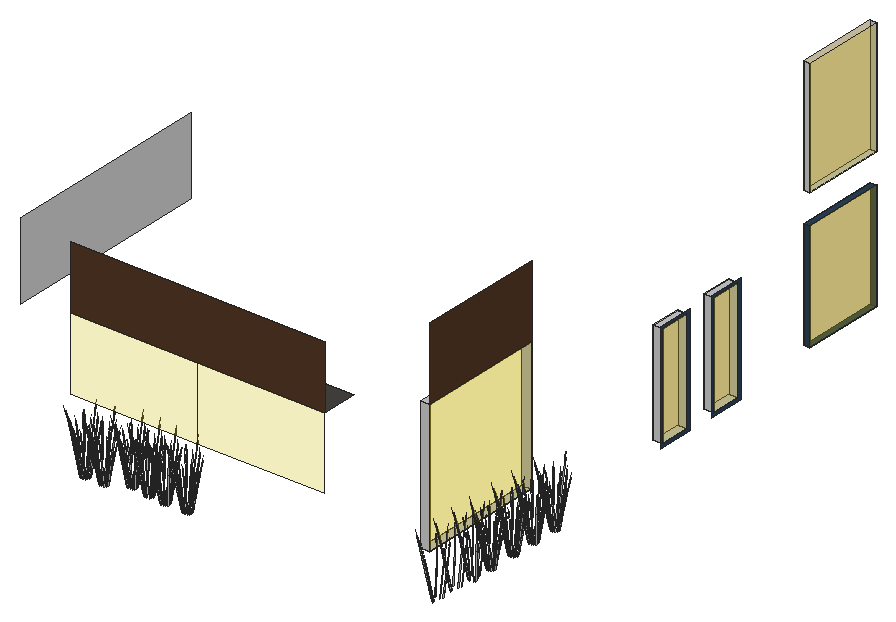
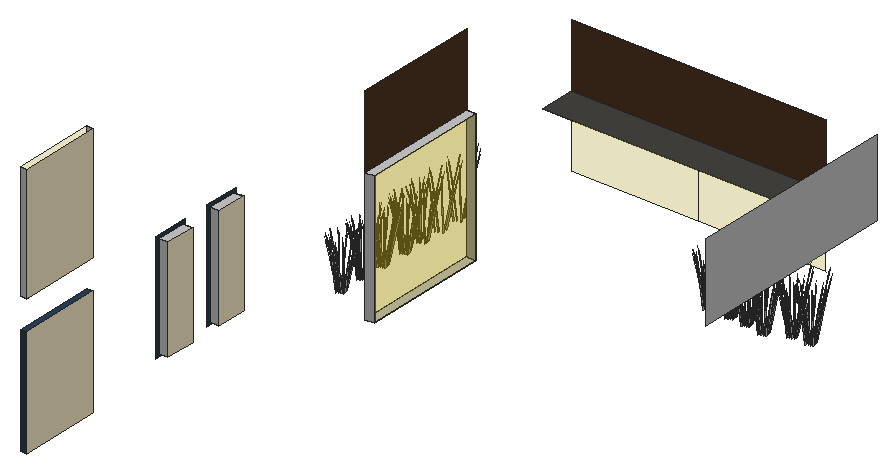
# SketchUp Ruby script. Lengths in inches.
U = 1.inch
M = Sketchup.active_model
def pt(a) = Geom::Point3d.new(a.map { |v| v * U })
def face(e, loops, mat)
  f = e.add_face(loops[0].map { |a| pt(a) })
  loops[1..].each { |l| e.add_face(l.map { |a| pt(a) }).erase! }
  f.material = f.back_material = mat if mat
  f
end
# faces: each face lists its corners as indices into pts; further lists are holes
def faces(e, pts, list, mat = nil) = list.each { |f| face(e, (f[0].is_a?(Array) ? f : [f]).map { |l| l.map { |i| pts[i] } }, mat) }
# xy, xz, yz: faces in a plane at the given z, y or x. An outline is a flat list of corners, or four numbers for a rectangle; further outlines are holes
def ring(l) = l.size == 4 ? [[l[0], l[1]], [l[2], l[1]], [l[2], l[3]], [l[0], l[3]]] : l.each_slice(2).to_a
def flat(e, list, mat, &to3) = list.each { |f| face(e, (f[0].is_a?(Array) ? f : [f]).map { |l| ring(l).map { |u, v| to3.(u, v) } }, mat) }
def xy(e, z, list, mat = nil) = flat(e, list, mat) { |x, y| [x, y, z] }
def xz(e, y, list, mat = nil) = flat(e, list, mat) { |x, z| [x, y, z] }
def yz(e, x, list, mat = nil) = flat(e, list, mat) { |y, z| [x, y, z] }
def lines(e, pts, list) = list.each { |a, b| e.add_line(pt(pts[a]), pt(pts[b])) }
# prism: a flat outline (further loops are holes) pulled along v
def prism(e, loops, v, mat = nil)
  f = face(e, loops, mat); d = Geom::Vector3d.new(v.map { |x| x * U })
  f.pushpull(f.normal.samedirection?(d) ? d.length : -d.length)
end
def box(e, o, s, mat = nil) = prism(e, [[o, [o[0] + s[0], o[1], o[2]], [o[0] + s[0], o[1] + s[1], o[2]], [o[0], o[1] + s[1], o[2]]]], [0, 0, s[2]], mat)
def at(x, y, z, deg = 0) = Geom::Transformation.translation(pt([x, y, z])) * Geom::Transformation.rotation(ORIGIN, Z_AXIS, deg.degrees)
def axes(o, x, y, z) = Geom::Transformation.new([*x, 0, *y, 0, *z, 0, *pt(o).to_a, 1])
def part(name) = M.definitions.add(name)
# library, detail: a bought-in or finely detailed component or shape, given as its bounding box
def library(name, o, s) = part(name).tap { |d| box(d.entities, o, s) }
def detail(e, o, s) = box(e.add_group.entities, o, s)
def put(e, d, t, mat = nil) = e.add_instance(d, t).tap { |i| i.material = mat if mat }
def group(e, t, mat = nil) = e.add_group.tap { |g| g.transformation = t; g.material = mat if mat }.entities
root = M.entities
M.materials.add("Carpet_04_1K").color = [43, 65, 85]
M.materials.add("D01_Frost_White").color = [255, 242, 206]
M.materials.add("Glass_Basic_01").color = [255, 228, 0]
M.materials["Glass_Basic_01"].alpha = 0.25
M.materials.add("LightPink_Translucent").color = [144, 107, 117]
M.materials["LightPink_Translucent"].alpha = 0.75
M.materials.add("Wood_Planks_01_1K").color = [69, 67, 63]
M.materials.add("Wood_Veneer_15_1K").color = [81, 54, 35]
M.materials.add("[_0053_Ivory_]").color = [200, 200, 200]
c1 = part("blade")
p = [[2.15,0.21,22],[0,0.17,0],[0.09,0.45,0],[2.18,0.31,22],[2.29,0.31,22],[0.38,0.45,0],
  [2.48,0.24,33],[2.49,0.24,33],[2.48,0.22,33]]
faces(c1.entities,p,[[0,1,2,3],[4,5,2,3],[6,3,4,7],[8,0,3,6]])
c2 = part("seeds")
p = [[0.3,-0.1,1.38],[-0.01,-0.03,1.59],[-0.01,-0.03,0.03],[0.14,-0.07,-0.07],[0.29,-0.03,3],[0.15,0.01,3.11]]
faces(c2.entities,p,[[0,1,2,3],[1,0,4,5]],"LightPink_Translucent")
c3 = part("blade with seeds")
put(c3.entities,c1,at(0,0,0))
put(c3.entities,c2,axes([2.4,0.25,30.99],[1.5799,-0.05474,1.17369],[-0.12525,1.92788,0.29478],[-0.07173,-0.02425,1.56792]))
xy(root,135,[[605.51,143.15,611.51,227.15]],"[_0053_Ivory_]")
xy(root,150,[[643.1,411.95,647.1,467.15]],"Carpet_04_1K")
xy(root,152,[[647.1,283.15,653.51,303.15],[647.1,325.15,653.51,345.15]],"[_0053_Ivory_]")
xy(root,220,[[647.1,283.15,653.51,303.15],[647.1,325.15,653.51,345.15]],"[_0053_Ivory_]")
xy(root,222,[[643.1,411.95,647.1,467.15]],"Carpet_04_1K")
xy(root,222,[[605.51,143.15,611.51,227.15]],"[_0053_Ivory_]")
xy(root,225,[[410.51,98.15,578.51,122.15]],"Wood_Planks_01_1K")
xy(root,241.75,[[643.1,411.95,647.1,467.15]],"[_0053_Ivory_]")
xz(root,98.15,[[410.51,177,494.51,225],[494.51,177,578.51,225]],"Glass_Basic_01")
xz(root,98.15,[[410.51,225,578.51,267]],"Wood_Veneer_15_1K")
xz(root,143.15,[[605.51,135,611.51,222]],"[_0053_Ivory_]")
xz(root,227.15,[[605.51,135,611.51,222]],"[_0053_Ivory_]")
xz(root,283.15,[[647.1,152,653.51,220]],"[_0053_Ivory_]")
xz(root,303.15,[[647.1,152,653.51,220]],"[_0053_Ivory_]")
xz(root,325.15,[[647.1,152,653.51,220]],"[_0053_Ivory_]")
xz(root,345.15,[[647.1,152,653.51,220]],"[_0053_Ivory_]")
xz(root,411.95,[[643.1,150,647.1,222]],"Carpet_04_1K")
xz(root,411.95,[[643.1,241.75,647.1,318]],"[_0053_Ivory_]")
xz(root,467.15,[[643.1,150,647.1,222]],"Carpet_04_1K")
xz(root,467.15,[[643.1,241.75,647.1,318]],"[_0053_Ivory_]")
yz(root,377.51,[[98.15,219,239.15,270]],"[_0053_Ivory_]")
yz(root,605.51,[[143.15,135,227.15,222]],"Glass_Basic_01")
yz(root,611.51,[[143.15,135,227.15,222]],"Glass_Basic_01")
yz(root,611.51,[[143.15,222,227.15,270]],"Wood_Veneer_15_1K")
yz(root,643.1,[[411.95,150,467.15,222],[411.95,241.75,467.15,318]],"D01_Frost_White")
yz(root,647.1,[[283.15,152,303.15,220],[325.15,152,345.15,220]],"D01_Frost_White")
yz(root,647.1,[[411.95,150,467.15,222],[411.95,241.75,467.15,318]],"Glass_Basic_01")
yz(root,653.51,[[[281.15,150,305.15,222],[283.15,152,303.15,220]],[[323.15,150,347.15,222],[325.15,152,345.15,220]]],"Carpet_04_1K")
yz(root,653.51,[[283.15,152,303.15,220],[325.15,152,345.15,220]],"Glass_Basic_01")
p = [[410.51,98.15,177],[410.43,98.15,177]]
lines(root,p,[[0,1]])
put(root,c3,axes([644.625,141.69,131.7],[-0.0938,-0.50652,0.35414],[0.53623,-0.13375,-0.4572],[0.14403,0.14515,0.87481]),"[_0053_Ivory_]")
put(root,c3,axes([646.18,138.67,131.7],[-0.52868,0.08987,0.35414],[-0.1396,-0.51376,-0.4572],[0.1515,-0.13799,0.87481]),"[_0053_Ivory_]")
put(root,c3,axes([641.39,138.97,131.7],[0.50475,0.17543,0.35414],[-0.14722,0.5118,-0.4572],[-0.20322,0.04693,0.87481]),"[_0053_Ivory_]")
put(root,c3,axes([645.46,137.65,131.7],[-0.41095,0.33109,0.35414],[-0.38901,-0.37805,-0.4572],[0.05919,-0.19208,0.87481]),"[_0053_Ivory_]")
put(root,c3,axes([643.03,137.1875,131.7],[0.0938,0.50652,0.35414],[-0.53623,0.13375,-0.4572],[-0.14403,-0.14515,0.87481]),"[_0053_Ivory_]")
put(root,c3,axes([643.34,156.05,131.7],[0.1831,-0.48359,0.35414],[0.53419,0.14105,-0.4572],[0.04898,0.1947,0.87481]),"[_0053_Ivory_]")
put(root,c3,axes([644.31,151.38,131.7],[-0.1831,0.48359,0.35414],[-0.53419,-0.14105,-0.4572],[-0.04898,-0.1947,0.87481]),"[_0053_Ivory_]")
put(root,c3,axes([645.69,155.28,131.7],[-0.34557,-0.39372,0.35414],[0.39459,-0.37271,-0.4572],[0.20048,0.05671,0.87481]),"[_0053_Ivory_]")
put(root,c3,axes([646.26,154.18,131.7],[-0.50475,-0.17543,0.35414],[0.14722,-0.5118,-0.4572],[0.20322,-0.04693,0.87481]),"[_0053_Ivory_]")
put(root,c3,axes([641.96,152.15,131.7],[0.34557,0.39372,0.35414],[-0.39459,0.37271,-0.4572],[-0.20048,-0.05671,0.87481]),"[_0053_Ivory_]")
put(root,c3,axes([642.1875,155.5,131.7],[0.41095,-0.33109,0.35414],[0.38901,0.37805,-0.4572],[-0.05919,0.19208,0.87481]),"[_0053_Ivory_]")
put(root,c3,axes([641.48,154.48,131.7],[0.52868,-0.08987,0.35414],[0.1396,0.51376,-0.4572],[-0.1515,0.13799,0.87481]),"[_0053_Ivory_]")
put(root,c3,axes([644.625,155.97,131.7],[-0.0938,-0.50652,0.35414],[0.53623,-0.13375,-0.4572],[0.14403,0.14515,0.87481]),"[_0053_Ivory_]")
put(root,c3,axes([646.18,152.95,131.7],[-0.52868,0.08987,0.35414],[-0.1396,-0.51376,-0.4572],[0.1515,-0.13799,0.87481]),"[_0053_Ivory_]")
put(root,c3,axes([641.39,153.25,131.7],[0.50475,0.17543,0.35414],[-0.14722,0.5118,-0.4572],[-0.20322,0.04693,0.87481]),"[_0053_Ivory_]")
put(root,c3,axes([645.46,151.93,131.7],[-0.41095,0.33109,0.35414],[-0.38901,-0.37805,-0.4572],[0.05919,-0.19208,0.87481]),"[_0053_Ivory_]")
put(root,c3,axes([643.03,151.46,131.7],[0.0938,0.50652,0.35414],[-0.53623,0.13375,-0.4572],[-0.14403,-0.14515,0.87481]),"[_0053_Ivory_]")
put(root,c3,axes([643.34,174.53,131.7],[0.1831,-0.48359,0.35414],[0.53419,0.14105,-0.4572],[0.04898,0.1947,0.87481]),"[_0053_Ivory_]")
put(root,c3,axes([644.31,169.87,131.7],[-0.1831,0.48359,0.35414],[-0.53419,-0.14105,-0.4572],[-0.04898,-0.1947,0.87481]),"[_0053_Ivory_]")
put(root,c3,axes([645.69,173.77,131.7],[-0.34557,-0.39372,0.35414],[0.39459,-0.37271,-0.4572],[0.20048,0.05671,0.87481]),"[_0053_Ivory_]")
put(root,c3,axes([646.26,172.66,131.7],[-0.50475,-0.17543,0.35414],[0.14722,-0.5118,-0.4572],[0.20322,-0.04693,0.87481]),"[_0053_Ivory_]")
put(root,c3,axes([641.96,170.63,131.7],[0.34557,0.39372,0.35414],[-0.39459,0.37271,-0.4572],[-0.20048,-0.05671,0.87481]),"[_0053_Ivory_]")
put(root,c3,axes([642.1875,173.99,131.7],[0.41095,-0.33109,0.35414],[0.38901,0.37805,-0.4572],[-0.05919,0.19208,0.87481]),"[_0053_Ivory_]")
put(root,c3,axes([641.48,172.96,131.7],[0.52868,-0.08987,0.35414],[0.1396,0.51376,-0.4572],[-0.1515,0.13799,0.87481]),"[_0053_Ivory_]")
put(root,c3,axes([644.625,174.45,131.7],[-0.0938,-0.50652,0.35414],[0.53623,-0.13375,-0.4572],[0.14403,0.14515,0.87481]),"[_0053_Ivory_]")
put(root,c3,axes([646.18,171.43,131.7],[-0.52868,0.08987,0.35414],[-0.1396,-0.51376,-0.4572],[0.1515,-0.13799,0.87481]),"[_0053_Ivory_]")
put(root,c3,axes([641.39,171.73,131.7],[0.50475,0.17543,0.35414],[-0.14722,0.5118,-0.4572],[-0.20322,0.04693,0.87481]),"[_0053_Ivory_]")
put(root,c3,axes([645.46,170.41,131.7],[-0.41095,0.33109,0.35414],[-0.38901,-0.37805,-0.4572],[0.05919,-0.19208,0.87481]),"[_0053_Ivory_]")
put(root,c3,axes([643.03,169.95,131.7],[0.0938,0.50652,0.35414],[-0.53623,0.13375,-0.4572],[-0.14403,-0.14515,0.87481]),"[_0053_Ivory_]")
put(root,c3,axes([643.34,191.29,131.7],[0.1831,-0.48359,0.35414],[0.53419,0.14105,-0.4572],[0.04898,0.1947,0.87481]),"[_0053_Ivory_]")
put(root,c3,axes([644.31,186.625,131.7],[-0.1831,0.48359,0.35414],[-0.53419,-0.14105,-0.4572],[-0.04898,-0.1947,0.87481]),"[_0053_Ivory_]")
put(root,c3,axes([645.69,190.53,131.7],[-0.34557,-0.39372,0.35414],[0.39459,-0.37271,-0.4572],[0.20048,0.05671,0.87481]),"[_0053_Ivory_]")
put(root,c3,axes([646.26,189.42,131.7],[-0.50475,-0.17543,0.35414],[0.14722,-0.5118,-0.4572],[0.20322,-0.04693,0.87481]),"[_0053_Ivory_]")
put(root,c3,axes([641.96,187.39,131.7],[0.34557,0.39372,0.35414],[-0.39459,0.37271,-0.4572],[-0.20048,-0.05671,0.87481]),"[_0053_Ivory_]")
put(root,c3,axes([642.1875,190.75,131.7],[0.41095,-0.33109,0.35414],[0.38901,0.37805,-0.4572],[-0.05919,0.19208,0.87481]),"[_0053_Ivory_]")
put(root,c3,axes([641.48,189.72,131.7],[0.52868,-0.08987,0.35414],[0.1396,0.51376,-0.4572],[-0.1515,0.13799,0.87481]),"[_0053_Ivory_]")
put(root,c3,axes([644.625,191.21,131.7],[-0.0938,-0.50652,0.35414],[0.53623,-0.13375,-0.4572],[0.14403,0.14515,0.87481]),"[_0053_Ivory_]")
put(root,c3,axes([646.18,188.19,131.7],[-0.52868,0.08987,0.35414],[-0.1396,-0.51376,-0.4572],[0.1515,-0.13799,0.87481]),"[_0053_Ivory_]")
put(root,c3,axes([641.39,188.49,131.7],[0.50475,0.17543,0.35414],[-0.14722,0.5118,-0.4572],[-0.20322,0.04693,0.87481]),"[_0053_Ivory_]")
put(root,c3,axes([645.46,187.17,131.7],[-0.41095,0.33109,0.35414],[-0.38901,-0.37805,-0.4572],[0.05919,-0.19208,0.87481]),"[_0053_Ivory_]")
put(root,c3,axes([643.03,186.71,131.7],[0.0938,0.50652,0.35414],[-0.53623,0.13375,-0.4572],[-0.14403,-0.14515,0.87481]),"[_0053_Ivory_]")
put(root,c3,axes([643.34,208.88,131.7],[0.1831,-0.48359,0.35414],[0.53419,0.14105,-0.4572],[0.04898,0.1947,0.87481]),"[_0053_Ivory_]")
put(root,c3,axes([644.31,204.22,131.7],[-0.1831,0.48359,0.35414],[-0.53419,-0.14105,-0.4572],[-0.04898,-0.1947,0.87481]),"[_0053_Ivory_]")
put(root,c3,axes([645.69,208.12,131.7],[-0.34557,-0.39372,0.35414],[0.39459,-0.37271,-0.4572],[0.20048,0.05671,0.87481]),"[_0053_Ivory_]")
put(root,c3,axes([646.26,207.01,131.7],[-0.50475,-0.17543,0.35414],[0.14722,-0.5118,-0.4572],[0.20322,-0.04693,0.87481]),"[_0053_Ivory_]")
put(root,c3,axes([641.96,204.98,131.7],[0.34557,0.39372,0.35414],[-0.39459,0.37271,-0.4572],[-0.20048,-0.05671,0.87481]),"[_0053_Ivory_]")
put(root,c3,axes([642.1875,208.34,131.7],[0.41095,-0.33109,0.35414],[0.38901,0.37805,-0.4572],[-0.05919,0.19208,0.87481]),"[_0053_Ivory_]")
put(root,c3,axes([641.48,207.3125,131.7],[0.52868,-0.08987,0.35414],[0.1396,0.51376,-0.4572],[-0.1515,0.13799,0.87481]),"[_0053_Ivory_]")
put(root,c3,axes([644.625,208.8,131.7],[-0.0938,-0.50652,0.35414],[0.53623,-0.13375,-0.4572],[0.14403,0.14515,0.87481]),"[_0053_Ivory_]")
put(root,c3,axes([646.18,205.78,131.7],[-0.52868,0.08987,0.35414],[-0.1396,-0.51376,-0.4572],[0.1515,-0.13799,0.87481]),"[_0053_Ivory_]")
put(root,c3,axes([641.39,206.08,131.7],[0.50475,0.17543,0.35414],[-0.14722,0.5118,-0.4572],[-0.20322,0.04693,0.87481]),"[_0053_Ivory_]")
put(root,c3,axes([645.46,204.76,131.7],[-0.41095,0.33109,0.35414],[-0.38901,-0.37805,-0.4572],[0.05919,-0.19208,0.87481]),"[_0053_Ivory_]")
put(root,c3,axes([643.03,204.3,131.7],[0.0938,0.50652,0.35414],[-0.53623,0.13375,-0.4572],[-0.14403,-0.14515,0.87481]),"[_0053_Ivory_]")
put(root,c3,axes([420,100.76,131.7],[0.1831,-0.48359,0.35414],[0.53419,0.14105,-0.4572],[0.04898,0.1947,0.87481]),"[_0053_Ivory_]")
put(root,c3,axes([420.97,96.09,131.7],[-0.1831,0.48359,0.35414],[-0.53419,-0.14105,-0.4572],[-0.04898,-0.1947,0.87481]),"[_0053_Ivory_]")
put(root,c3,axes([422.35,99.99,131.7],[-0.34557,-0.39372,0.35414],[0.39459,-0.37271,-0.4572],[0.20048,0.05671,0.87481]),"[_0053_Ivory_]")
put(root,c3,axes([422.92,98.89,131.7],[-0.50475,-0.17543,0.35414],[0.14722,-0.5118,-0.4572],[0.20322,-0.04693,0.87481]),"[_0053_Ivory_]")
put(root,c3,axes([418.62,96.86,131.7],[0.34557,0.39372,0.35414],[-0.39459,0.37271,-0.4572],[-0.20048,-0.05671,0.87481]),"[_0053_Ivory_]")
put(root,c3,axes([418.85,100.21,131.7],[0.41095,-0.33109,0.35414],[0.38901,0.37805,-0.4572],[-0.05919,0.19208,0.87481]),"[_0053_Ivory_]")
put(root,c3,axes([418.13,99.1875,131.7],[0.52868,-0.08987,0.35414],[0.1396,0.51376,-0.4572],[-0.1515,0.13799,0.87481]),"[_0053_Ivory_]")
put(root,c3,axes([421.28,100.68,131.7],[-0.0938,-0.50652,0.35414],[0.53623,-0.13375,-0.4572],[0.14403,0.14515,0.87481]),"[_0053_Ivory_]")
put(root,c3,axes([422.84,97.66,131.7],[-0.52868,0.08987,0.35414],[-0.1396,-0.51376,-0.4572],[0.1515,-0.13799,0.87481]),"[_0053_Ivory_]")
put(root,c3,axes([418.05,97.96,131.7],[0.50475,0.17543,0.35414],[-0.14722,0.5118,-0.4572],[-0.20322,0.04693,0.87481]),"[_0053_Ivory_]")
put(root,c3,axes([422.12,96.64,131.7],[-0.41095,0.33109,0.35414],[-0.38901,-0.37805,-0.4572],[0.05919,-0.19208,0.87481]),"[_0053_Ivory_]")
put(root,c3,axes([419.6875,96.17,131.7],[0.0938,0.50652,0.35414],[-0.53623,0.13375,-0.4572],[-0.14403,-0.14515,0.87481]),"[_0053_Ivory_]")
put(root,c3,axes([432.22,100.76,131.7],[0.1831,-0.48359,0.35414],[0.53419,0.14105,-0.4572],[0.04898,0.1947,0.87481]),"[_0053_Ivory_]")
put(root,c3,axes([433.18,96.09,131.7],[-0.1831,0.48359,0.35414],[-0.53419,-0.14105,-0.4572],[-0.04898,-0.1947,0.87481]),"[_0053_Ivory_]")
put(root,c3,axes([434.57,99.99,131.7],[-0.34557,-0.39372,0.35414],[0.39459,-0.37271,-0.4572],[0.20048,0.05671,0.87481]),"[_0053_Ivory_]")
put(root,c3,axes([435.13,98.89,131.7],[-0.50475,-0.17543,0.35414],[0.14722,-0.5118,-0.4572],[0.20322,-0.04693,0.87481]),"[_0053_Ivory_]")
put(root,c3,axes([430.83,96.86,131.7],[0.34557,0.39372,0.35414],[-0.39459,0.37271,-0.4572],[-0.20048,-0.05671,0.87481]),"[_0053_Ivory_]")
put(root,c3,axes([431.0625,100.21,131.7],[0.41095,-0.33109,0.35414],[0.38901,0.37805,-0.4572],[-0.05919,0.19208,0.87481]),"[_0053_Ivory_]")
put(root,c3,axes([430.35,99.1875,131.7],[0.52868,-0.08987,0.35414],[0.1396,0.51376,-0.4572],[-0.1515,0.13799,0.87481]),"[_0053_Ivory_]")
put(root,c3,axes([433.5,100.68,131.7],[-0.0938,-0.50652,0.35414],[0.53623,-0.13375,-0.4572],[0.14403,0.14515,0.87481]),"[_0053_Ivory_]")
put(root,c3,axes([435.05,97.66,131.7],[-0.52868,0.08987,0.35414],[-0.1396,-0.51376,-0.4572],[0.1515,-0.13799,0.87481]),"[_0053_Ivory_]")
put(root,c3,axes([430.26,97.96,131.7],[0.50475,0.17543,0.35414],[-0.14722,0.5118,-0.4572],[-0.20322,0.04693,0.87481]),"[_0053_Ivory_]")
put(root,c3,axes([434.34,96.64,131.7],[-0.41095,0.33109,0.35414],[-0.38901,-0.37805,-0.4572],[0.05919,-0.19208,0.87481]),"[_0053_Ivory_]")
put(root,c3,axes([431.9,96.17,131.7],[0.0938,0.50652,0.35414],[-0.53623,0.13375,-0.4572],[-0.14403,-0.14515,0.87481]),"[_0053_Ivory_]")
put(root,c3,axes([445.62,107.57,131.7],[0.1831,-0.48359,0.35414],[0.53419,0.14105,-0.4572],[0.04898,0.1947,0.87481]),"[_0053_Ivory_]")
put(root,c3,axes([446.59,102.9,131.7],[-0.1831,0.48359,0.35414],[-0.53419,-0.14105,-0.4572],[-0.04898,-0.1947,0.87481]),"[_0053_Ivory_]")
put(root,c3,axes([447.97,106.8,131.7],[-0.34557,-0.39372,0.35414],[0.39459,-0.37271,-0.4572],[0.20048,0.05671,0.87481]),"[_0053_Ivory_]")
put(root,c3,axes([448.54,105.7,131.7],[-0.50475,-0.17543,0.35414],[0.14722,-0.5118,-0.4572],[0.20322,-0.04693,0.87481]),"[_0053_Ivory_]")
put(root,c3,axes([444.24,103.67,131.7],[0.34557,0.39372,0.35414],[-0.39459,0.37271,-0.4572],[-0.20048,-0.05671,0.87481]),"[_0053_Ivory_]")
put(root,c3,axes([444.47,107.02,131.7],[0.41095,-0.33109,0.35414],[0.38901,0.37805,-0.4572],[-0.05919,0.19208,0.87481]),"[_0053_Ivory_]")
put(root,c3,axes([443.75,106,131.7],[0.52868,-0.08987,0.35414],[0.1396,0.51376,-0.4572],[-0.1515,0.13799,0.87481]),"[_0053_Ivory_]")
put(root,c3,axes([446.9,107.49,131.7],[-0.0938,-0.50652,0.35414],[0.53623,-0.13375,-0.4572],[0.14403,0.14515,0.87481]),"[_0053_Ivory_]")
put(root,c3,axes([448.45,104.47,131.7],[-0.52868,0.08987,0.35414],[-0.1396,-0.51376,-0.4572],[0.1515,-0.13799,0.87481]),"[_0053_Ivory_]")
put(root,c3,axes([443.67,104.77,131.7],[0.50475,0.17543,0.35414],[-0.14722,0.5118,-0.4572],[-0.20322,0.04693,0.87481]),"[_0053_Ivory_]")
put(root,c3,axes([447.74,103.45,131.7],[-0.41095,0.33109,0.35414],[-0.38901,-0.37805,-0.4572],[0.05919,-0.19208,0.87481]),"[_0053_Ivory_]")
put(root,c3,axes([445.3,102.98,131.7],[0.0938,0.50652,0.35414],[-0.53623,0.13375,-0.4572],[-0.14403,-0.14515,0.87481]),"[_0053_Ivory_]")
put(root,c3,axes([458.1,105.75,131.7],[0.1831,-0.48359,0.35414],[0.53419,0.14105,-0.4572],[0.04898,0.1947,0.87481]),"[_0053_Ivory_]")
put(root,c3,axes([459.07,101.08,131.7],[-0.1831,0.48359,0.35414],[-0.53419,-0.14105,-0.4572],[-0.04898,-0.1947,0.87481]),"[_0053_Ivory_]")
put(root,c3,axes([460.45,104.98,131.7],[-0.34557,-0.39372,0.35414],[0.39459,-0.37271,-0.4572],[0.20048,0.05671,0.87481]),"[_0053_Ivory_]")
put(root,c3,axes([461.02,103.88,131.7],[-0.50475,-0.17543,0.35414],[0.14722,-0.5118,-0.4572],[0.20322,-0.04693,0.87481]),"[_0053_Ivory_]")
put(root,c3,axes([456.72,101.85,131.7],[0.34557,0.39372,0.35414],[-0.39459,0.37271,-0.4572],[-0.20048,-0.05671,0.87481]),"[_0053_Ivory_]")
put(root,c3,axes([456.95,105.2,131.7],[0.41095,-0.33109,0.35414],[0.38901,0.37805,-0.4572],[-0.05919,0.19208,0.87481]),"[_0053_Ivory_]")
put(root,c3,axes([456.23,104.18,131.7],[0.52868,-0.08987,0.35414],[0.1396,0.51376,-0.4572],[-0.1515,0.13799,0.87481]),"[_0053_Ivory_]")
put(root,c3,axes([459.38,105.67,131.7],[-0.0938,-0.50652,0.35414],[0.53623,-0.13375,-0.4572],[0.14403,0.14515,0.87481]),"[_0053_Ivory_]")
put(root,c3,axes([460.94,102.65,131.7],[-0.52868,0.08987,0.35414],[-0.1396,-0.51376,-0.4572],[0.1515,-0.13799,0.87481]),"[_0053_Ivory_]")
put(root,c3,axes([456.15,102.95,131.7],[0.50475,0.17543,0.35414],[-0.14722,0.5118,-0.4572],[-0.20322,0.04693,0.87481]),"[_0053_Ivory_]")
put(root,c3,axes([460.22,101.63,131.7],[-0.41095,0.33109,0.35414],[-0.38901,-0.37805,-0.4572],[0.05919,-0.19208,0.87481]),"[_0053_Ivory_]")
put(root,c3,axes([457.79,101.16,131.7],[0.0938,0.50652,0.35414],[-0.53623,0.13375,-0.4572],[-0.14403,-0.14515,0.87481]),"[_0053_Ivory_]")
put(root,c3,axes([469.61,104.89,131.7],[0.1831,-0.48359,0.35414],[0.53419,0.14105,-0.4572],[0.04898,0.1947,0.87481]),"[_0053_Ivory_]")
put(root,c3,axes([470.58,100.23,131.7],[-0.1831,0.48359,0.35414],[-0.53419,-0.14105,-0.4572],[-0.04898,-0.1947,0.87481]),"[_0053_Ivory_]")
put(root,c3,axes([471.96,104.125,131.7],[-0.34557,-0.39372,0.35414],[0.39459,-0.37271,-0.4572],[0.20048,0.05671,0.87481]),"[_0053_Ivory_]")
put(root,c3,axes([472.53,103.02,131.7],[-0.50475,-0.17543,0.35414],[0.14722,-0.5118,-0.4572],[0.20322,-0.04693,0.87481]),"[_0053_Ivory_]")
put(root,c3,axes([468.23,100.99,131.7],[0.34557,0.39372,0.35414],[-0.39459,0.37271,-0.4572],[-0.20048,-0.05671,0.87481]),"[_0053_Ivory_]")
put(root,c3,axes([468.46,104.35,131.7],[0.41095,-0.33109,0.35414],[0.38901,0.37805,-0.4572],[-0.05919,0.19208,0.87481]),"[_0053_Ivory_]")
put(root,c3,axes([467.75,103.32,131.7],[0.52868,-0.08987,0.35414],[0.1396,0.51376,-0.4572],[-0.1515,0.13799,0.87481]),"[_0053_Ivory_]")
put(root,c3,axes([470.9,104.8125,131.7],[-0.0938,-0.50652,0.35414],[0.53623,-0.13375,-0.4572],[0.14403,0.14515,0.87481]),"[_0053_Ivory_]")
put(root,c3,axes([472.45,101.79,131.7],[-0.52868,0.08987,0.35414],[-0.1396,-0.51376,-0.4572],[0.1515,-0.13799,0.87481]),"[_0053_Ivory_]")
put(root,c3,axes([467.66,102.09,131.7],[0.50475,0.17543,0.35414],[-0.14722,0.5118,-0.4572],[-0.20322,0.04693,0.87481]),"[_0053_Ivory_]")
put(root,c3,axes([471.74,100.77,131.7],[-0.41095,0.33109,0.35414],[-0.38901,-0.37805,-0.4572],[0.05919,-0.19208,0.87481]),"[_0053_Ivory_]")
put(root,c3,axes([469.3,100.31,131.7],[0.0938,0.50652,0.35414],[-0.53623,0.13375,-0.4572],[-0.14403,-0.14515,0.87481]),"[_0053_Ivory_]")
put(root,c3,axes([484.11,104.68,131.7],[0.1831,-0.48359,0.35414],[0.53419,0.14105,-0.4572],[0.04898,0.1947,0.87481]),"[_0053_Ivory_]")
put(root,c3,axes([485.07,100.02,131.7],[-0.1831,0.48359,0.35414],[-0.53419,-0.14105,-0.4572],[-0.04898,-0.1947,0.87481]),"[_0053_Ivory_]")
put(root,c3,axes([486.46,103.92,131.7],[-0.34557,-0.39372,0.35414],[0.39459,-0.37271,-0.4572],[0.20048,0.05671,0.87481]),"[_0053_Ivory_]")
put(root,c3,axes([487.02,102.8125,131.7],[-0.50475,-0.17543,0.35414],[0.14722,-0.5118,-0.4572],[0.20322,-0.04693,0.87481]),"[_0053_Ivory_]")
put(root,c3,axes([482.72,100.78,131.7],[0.34557,0.39372,0.35414],[-0.39459,0.37271,-0.4572],[-0.20048,-0.05671,0.87481]),"[_0053_Ivory_]")
put(root,c3,axes([482.95,104.14,131.7],[0.41095,-0.33109,0.35414],[0.38901,0.37805,-0.4572],[-0.05919,0.19208,0.87481]),"[_0053_Ivory_]")
put(root,c3,axes([482.24,103.11,131.7],[0.52868,-0.08987,0.35414],[0.1396,0.51376,-0.4572],[-0.1515,0.13799,0.87481]),"[_0053_Ivory_]")
put(root,c3,axes([485.39,104.6,131.7],[-0.0938,-0.50652,0.35414],[0.53623,-0.13375,-0.4572],[0.14403,0.14515,0.87481]),"[_0053_Ivory_]")
put(root,c3,axes([486.94,101.58,131.7],[-0.52868,0.08987,0.35414],[-0.1396,-0.51376,-0.4572],[0.1515,-0.13799,0.87481]),"[_0053_Ivory_]")
put(root,c3,axes([482.15,101.88,131.7],[0.50475,0.17543,0.35414],[-0.14722,0.5118,-0.4572],[-0.20322,0.04693,0.87481]),"[_0053_Ivory_]")
put(root,c3,axes([486.23,100.5625,131.7],[-0.41095,0.33109,0.35414],[-0.38901,-0.37805,-0.4572],[0.05919,-0.19208,0.87481]),"[_0053_Ivory_]")
put(root,c3,axes([483.79,100.1,131.7],[0.0938,0.50652,0.35414],[-0.53623,0.13375,-0.4572],[-0.14403,-0.14515,0.87481]),"[_0053_Ivory_]")
put(root,c3,axes([643.33,112.1875,131.72],[-0.59846,-0.1644,0.53283],[0.20464,-0.54049,0.43934],[0.03596,0.21255,1.10256]),"[_0053_Ivory_]")
put(root,c3,axes([643.33,127.25,131.72],[-0.59846,-0.1644,0.53283],[0.20464,-0.54049,0.43934],[0.03596,0.21255,1.10256]),"[_0053_Ivory_]")
put(root,c3,axes([643.33,142.17,131.72],[-0.59846,-0.1644,0.53283],[0.20464,-0.54049,0.43934],[0.03596,0.21255,1.10256]),"[_0053_Ivory_]")
put(root,c3,axes([643.33,156.44,131.72],[-0.59846,-0.1644,0.53283],[0.20464,-0.54049,0.43934],[0.03596,0.21255,1.10256]),"[_0053_Ivory_]")
put(root,c3,axes([643.33,174.93,131.72],[-0.59846,-0.1644,0.53283],[0.20464,-0.54049,0.43934],[0.03596,0.21255,1.10256]),"[_0053_Ivory_]")
put(root,c3,axes([643.33,191.6875,131.72],[-0.59846,-0.1644,0.53283],[0.20464,-0.54049,0.43934],[0.03596,0.21255,1.10256]),"[_0053_Ivory_]")
put(root,c3,axes([643.33,209.28,131.72],[-0.59846,-0.1644,0.53283],[0.20464,-0.54049,0.43934],[0.03596,0.21255,1.10256]),"[_0053_Ivory_]")
put(root,c3,axes([419.99,101.15,131.72],[-0.59846,-0.1644,0.53283],[0.20464,-0.54049,0.43934],[0.03596,0.21255,1.10256]),"[_0053_Ivory_]")
put(root,c3,axes([432.21,101.15,131.72],[-0.59846,-0.1644,0.53283],[0.20464,-0.54049,0.43934],[0.03596,0.21255,1.10256]),"[_0053_Ivory_]")
put(root,c3,axes([445.61,107.96,131.72],[-0.59846,-0.1644,0.53283],[0.20464,-0.54049,0.43934],[0.03596,0.21255,1.10256]),"[_0053_Ivory_]")
put(root,c3,axes([458.09,106.15,131.72],[-0.59846,-0.1644,0.53283],[0.20464,-0.54049,0.43934],[0.03596,0.21255,1.10256]),"[_0053_Ivory_]")
put(root,c3,axes([469.61,105.29,131.72],[-0.59846,-0.1644,0.53283],[0.20464,-0.54049,0.43934],[0.03596,0.21255,1.10256]),"[_0053_Ivory_]")
put(root,c3,axes([484.1,105.08,131.72],[-0.59846,-0.1644,0.53283],[0.20464,-0.54049,0.43934],[0.03596,0.21255,1.10256]),"[_0053_Ivory_]")
put(root,c3,axes([641.42,107.54,131.75],[0.50157,-0.46409,0.53763],[0.43258,0.49285,0.4433],[-0.23532,-0.08561,1.11249]),"[_0053_Ivory_]")
put(root,c3,axes([642.79,106.61,131.75],[0.67657,-0.16163,0.53763],[0.11742,0.63404,0.4433],[-0.15912,-0.18687,1.11249]),"[_0053_Ivory_]")
put(root,c3,axes([641.42,122.6,131.75],[0.50157,-0.46409,0.53763],[0.43258,0.49285,0.4433],[-0.23532,-0.08561,1.11249]),"[_0053_Ivory_]")
put(root,c3,axes([642.79,121.67,131.75],[0.67657,-0.16163,0.53763],[0.11742,0.63404,0.4433],[-0.15912,-0.18687,1.11249]),"[_0053_Ivory_]")
put(root,c3,axes([641.42,137.52,131.75],[0.50157,-0.46409,0.53763],[0.43258,0.49285,0.4433],[-0.23532,-0.08561,1.11249]),"[_0053_Ivory_]")
put(root,c3,axes([642.79,136.59,131.75],[0.67657,-0.16163,0.53763],[0.11742,0.63404,0.4433],[-0.15912,-0.18687,1.11249]),"[_0053_Ivory_]")
put(root,c3,axes([641.42,151.79,131.75],[0.50157,-0.46409,0.53763],[0.43258,0.49285,0.4433],[-0.23532,-0.08561,1.11249]),"[_0053_Ivory_]")
put(root,c3,axes([642.79,150.87,131.75],[0.67657,-0.16163,0.53763],[0.11742,0.63404,0.4433],[-0.15912,-0.18687,1.11249]),"[_0053_Ivory_]")
put(root,c3,axes([641.42,170.28,131.75],[0.50157,-0.46409,0.53763],[0.43258,0.49285,0.4433],[-0.23532,-0.08561,1.11249]),"[_0053_Ivory_]")
put(root,c3,axes([642.79,169.35,131.75],[0.67657,-0.16163,0.53763],[0.11742,0.63404,0.4433],[-0.15912,-0.18687,1.11249]),"[_0053_Ivory_]")
put(root,c3,axes([641.42,187.04,131.75],[0.50157,-0.46409,0.53763],[0.43258,0.49285,0.4433],[-0.23532,-0.08561,1.11249]),"[_0053_Ivory_]")
put(root,c3,axes([642.79,186.11,131.75],[0.67657,-0.16163,0.53763],[0.11742,0.63404,0.4433],[-0.15912,-0.18687,1.11249]),"[_0053_Ivory_]")
put(root,c3,axes([641.42,204.625,131.75],[0.50157,-0.46409,0.53763],[0.43258,0.49285,0.4433],[-0.23532,-0.08561,1.11249]),"[_0053_Ivory_]")
put(root,c3,axes([642.79,203.7,131.75],[0.67657,-0.16163,0.53763],[0.11742,0.63404,0.4433],[-0.15912,-0.18687,1.11249]),"[_0053_Ivory_]")
put(root,c3,axes([418.08,96.5,131.75],[0.50157,-0.46409,0.53763],[0.43258,0.49285,0.4433],[-0.23532,-0.08561,1.11249]),"[_0053_Ivory_]")
put(root,c3,axes([419.45,95.58,131.75],[0.67657,-0.16163,0.53763],[0.11742,0.63404,0.4433],[-0.15912,-0.18687,1.11249]),"[_0053_Ivory_]")
put(root,c3,axes([430.29,96.5,131.75],[0.50157,-0.46409,0.53763],[0.43258,0.49285,0.4433],[-0.23532,-0.08561,1.11249]),"[_0053_Ivory_]")
put(root,c3,axes([431.66,95.58,131.75],[0.67657,-0.16163,0.53763],[0.11742,0.63404,0.4433],[-0.15912,-0.18687,1.11249]),"[_0053_Ivory_]")
put(root,c3,axes([443.69,103.3125,131.75],[0.50157,-0.46409,0.53763],[0.43258,0.49285,0.4433],[-0.23532,-0.08561,1.11249]),"[_0053_Ivory_]")
put(root,c3,axes([445.0625,102.39,131.75],[0.67657,-0.16163,0.53763],[0.11742,0.63404,0.4433],[-0.15912,-0.18687,1.11249]),"[_0053_Ivory_]")
put(root,c3,axes([456.18,101.49,131.75],[0.50157,-0.46409,0.53763],[0.43258,0.49285,0.4433],[-0.23532,-0.08561,1.11249]),"[_0053_Ivory_]")
put(root,c3,axes([457.55,100.57,131.75],[0.67657,-0.16163,0.53763],[0.11742,0.63404,0.4433],[-0.15912,-0.18687,1.11249]),"[_0053_Ivory_]")
put(root,c3,axes([467.69,100.64,131.75],[0.50157,-0.46409,0.53763],[0.43258,0.49285,0.4433],[-0.23532,-0.08561,1.11249]),"[_0053_Ivory_]")
put(root,c3,axes([469.06,99.71,131.75],[0.67657,-0.16163,0.53763],[0.11742,0.63404,0.4433],[-0.15912,-0.18687,1.11249]),"[_0053_Ivory_]")
put(root,c3,axes([482.18,100.43,131.75],[0.50157,-0.46409,0.53763],[0.43258,0.49285,0.4433],[-0.23532,-0.08561,1.11249]),"[_0053_Ivory_]")
put(root,c3,axes([483.55,99.5,131.75],[0.67657,-0.16163,0.53763],[0.11742,0.63404,0.4433],[-0.15912,-0.18687,1.11249]),"[_0053_Ivory_]")
put(root,c3,axes([644.06,113.52,132.3],[0.4197,-0.36076,-0.06488],[0.38456,0.39511,-0.29416],[0.02707,0.11196,0.97024]),"[_0053_Ivory_]")
put(root,c3,axes([640.28,111.68,132.3],[0.53595,0.16786,-0.06488],[-0.16486,0.51664,-0.29416],[-0.08766,0.07844,0.97024]),"[_0053_Ivory_]")
put(root,c3,axes([644.06,128.58,132.3],[0.4197,-0.36076,-0.06488],[0.38456,0.39511,-0.29416],[0.02707,0.11196,0.97024]),"[_0053_Ivory_]")
put(root,c3,axes([640.28,126.75,132.3],[0.53595,0.16786,-0.06488],[-0.16486,0.51664,-0.29416],[-0.08766,0.07844,0.97024]),"[_0053_Ivory_]")
put(root,c3,axes([644.06,143.5,132.3],[0.4197,-0.36076,-0.06488],[0.38456,0.39511,-0.29416],[0.02707,0.11196,0.97024]),"[_0053_Ivory_]")
put(root,c3,axes([640.28,141.66,132.3],[0.53595,0.16786,-0.06488],[-0.16486,0.51664,-0.29416],[-0.08766,0.07844,0.97024]),"[_0053_Ivory_]")
put(root,c3,axes([644.06,157.77,132.3],[0.4197,-0.36076,-0.06488],[0.38456,0.39511,-0.29416],[0.02707,0.11196,0.97024]),"[_0053_Ivory_]")
put(root,c3,axes([640.28,155.9375,132.3],[0.53595,0.16786,-0.06488],[-0.16486,0.51664,-0.29416],[-0.08766,0.07844,0.97024]),"[_0053_Ivory_]")
put(root,c3,axes([644.06,176.26,132.3],[0.4197,-0.36076,-0.06488],[0.38456,0.39511,-0.29416],[0.02707,0.11196,0.97024]),"[_0053_Ivory_]")
put(root,c3,axes([640.28,174.42,132.3],[0.53595,0.16786,-0.06488],[-0.16486,0.51664,-0.29416],[-0.08766,0.07844,0.97024]),"[_0053_Ivory_]")
put(root,c3,axes([644.06,193.02,132.3],[0.4197,-0.36076,-0.06488],[0.38456,0.39511,-0.29416],[0.02707,0.11196,0.97024]),"[_0053_Ivory_]")
put(root,c3,axes([640.28,191.18,132.3],[0.53595,0.16786,-0.06488],[-0.16486,0.51664,-0.29416],[-0.08766,0.07844,0.97024]),"[_0053_Ivory_]")
put(root,c3,axes([644.06,210.61,132.3],[0.4197,-0.36076,-0.06488],[0.38456,0.39511,-0.29416],[0.02707,0.11196,0.97024]),"[_0053_Ivory_]")
put(root,c3,axes([640.28,208.77,132.3],[0.53595,0.16786,-0.06488],[-0.16486,0.51664,-0.29416],[-0.08766,0.07844,0.97024]),"[_0053_Ivory_]")
put(root,c3,axes([420.72,102.48,132.3],[0.4197,-0.36076,-0.06488],[0.38456,0.39511,-0.29416],[0.02707,0.11196,0.97024]),"[_0053_Ivory_]")
put(root,c3,axes([416.93,100.65,132.3],[0.53595,0.16786,-0.06488],[-0.16486,0.51664,-0.29416],[-0.08766,0.07844,0.97024]),"[_0053_Ivory_]")
put(root,c3,axes([432.93,102.48,132.3],[0.4197,-0.36076,-0.06488],[0.38456,0.39511,-0.29416],[0.02707,0.11196,0.97024]),"[_0053_Ivory_]")
put(root,c3,axes([429.15,100.65,132.3],[0.53595,0.16786,-0.06488],[-0.16486,0.51664,-0.29416],[-0.08766,0.07844,0.97024]),"[_0053_Ivory_]")
put(root,c3,axes([446.34,109.29,132.3],[0.4197,-0.36076,-0.06488],[0.38456,0.39511,-0.29416],[0.02707,0.11196,0.97024]),"[_0053_Ivory_]")
put(root,c3,axes([442.55,107.46,132.3],[0.53595,0.16786,-0.06488],[-0.16486,0.51664,-0.29416],[-0.08766,0.07844,0.97024]),"[_0053_Ivory_]")
put(root,c3,axes([458.82,107.47,132.3],[0.4197,-0.36076,-0.06488],[0.38456,0.39511,-0.29416],[0.02707,0.11196,0.97024]),"[_0053_Ivory_]")
put(root,c3,axes([455.03,105.64,132.3],[0.53595,0.16786,-0.06488],[-0.16486,0.51664,-0.29416],[-0.08766,0.07844,0.97024]),"[_0053_Ivory_]")
put(root,c3,axes([470.33,106.62,132.3],[0.4197,-0.36076,-0.06488],[0.38456,0.39511,-0.29416],[0.02707,0.11196,0.97024]),"[_0053_Ivory_]")
put(root,c3,axes([466.55,104.78,132.3],[0.53595,0.16786,-0.06488],[-0.16486,0.51664,-0.29416],[-0.08766,0.07844,0.97024]),"[_0053_Ivory_]")
put(root,c3,axes([484.82,106.41,132.3],[0.4197,-0.36076,-0.06488],[0.38456,0.39511,-0.29416],[0.02707,0.11196,0.97024]),"[_0053_Ivory_]")
put(root,c3,axes([481.04,104.57,132.3],[0.53595,0.16786,-0.06488],[-0.16486,0.51664,-0.29416],[-0.08766,0.07844,0.97024]),"[_0053_Ivory_]")
